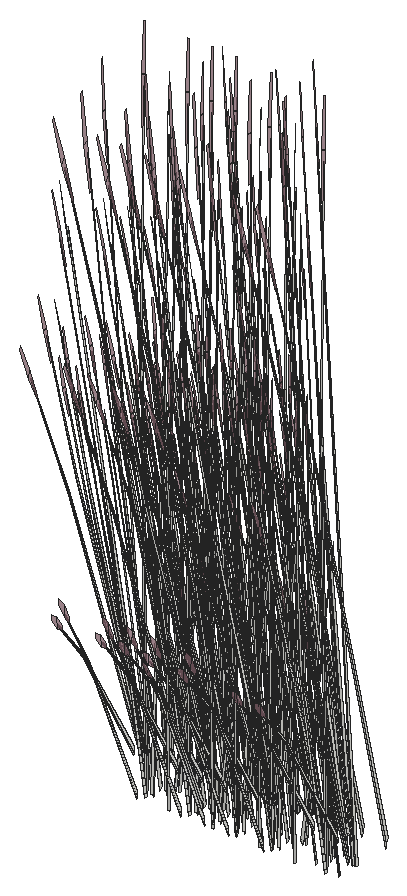
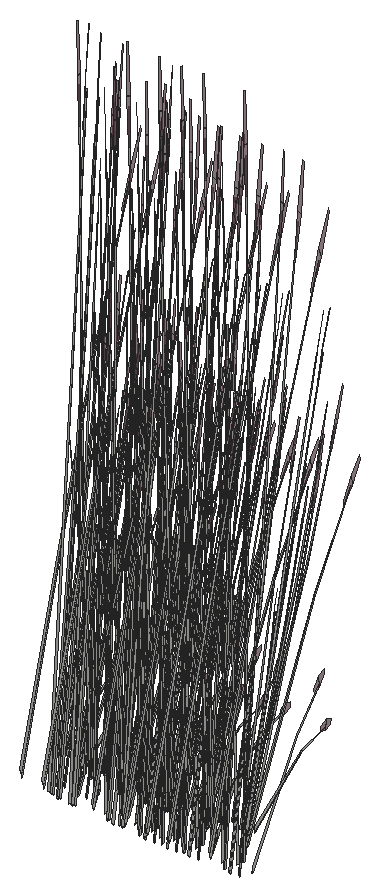
# SketchUp Ruby script. Lengths in inches.
U = 1.inch
M = Sketchup.active_model
def pt(a) = Geom::Point3d.new(a.map { |v| v * U })
def face(e, loops, mat)
  f = e.add_face(loops[0].map { |a| pt(a) })
  loops[1..].each { |l| e.add_face(l.map { |a| pt(a) }).erase! }
  f.material = f.back_material = mat if mat
  f
end
# faces: each face lists its corners as indices into pts; further lists are holes
def faces(e, pts, list, mat = nil) = list.each { |f| face(e, (f[0].is_a?(Array) ? f : [f]).map { |l| l.map { |i| pts[i] } }, mat) }
# xy, xz, yz: faces in a plane at the given z, y or x. An outline is a flat list of corners, or four numbers for a rectangle; further outlines are holes
def ring(l) = l.size == 4 ? [[l[0], l[1]], [l[2], l[1]], [l[2], l[3]], [l[0], l[3]]] : l.each_slice(2).to_a
def flat(e, list, mat, &to3) = list.each { |f| face(e, (f[0].is_a?(Array) ? f : [f]).map { |l| ring(l).map { |u, v| to3.(u, v) } }, mat) }
def xy(e, z, list, mat = nil) = flat(e, list, mat) { |x, y| [x, y, z] }
def xz(e, y, list, mat = nil) = flat(e, list, mat) { |x, z| [x, y, z] }
def yz(e, x, list, mat = nil) = flat(e, list, mat) { |y, z| [x, y, z] }
def lines(e, pts, list) = list.each { |a, b| e.add_line(pt(pts[a]), pt(pts[b])) }
# prism: a flat outline (further loops are holes) pulled along v
def prism(e, loops, v, mat = nil)
  f = face(e, loops, mat); d = Geom::Vector3d.new(v.map { |x| x * U })
  f.pushpull(f.normal.samedirection?(d) ? d.length : -d.length)
end
def box(e, o, s, mat = nil) = prism(e, [[o, [o[0] + s[0], o[1], o[2]], [o[0] + s[0], o[1] + s[1], o[2]], [o[0], o[1] + s[1], o[2]]]], [0, 0, s[2]], mat)
def at(x, y, z, deg = 0) = Geom::Transformation.translation(pt([x, y, z])) * Geom::Transformation.rotation(ORIGIN, Z_AXIS, deg.degrees)
def axes(o, x, y, z) = Geom::Transformation.new([*x, 0, *y, 0, *z, 0, *pt(o).to_a, 1])
def part(name) = M.definitions.add(name)
# library, detail: a bought-in or finely detailed component or shape, given as its bounding box
def library(name, o, s) = part(name).tap { |d| box(d.entities, o, s) }
def detail(e, o, s) = box(e.add_group.entities, o, s)
def put(e, d, t, mat = nil) = e.add_instance(d, t).tap { |i| i.material = mat if mat }
def group(e, t, mat = nil) = e.add_group.tap { |g| g.transformation = t; g.material = mat if mat }.entities
root = M.entities
M.materials.add("LightPink_Translucent").color = [144, 107, 117]
M.materials["LightPink_Translucent"].alpha = 0.75
c1 = part("blade")
p = [[2.15,0.21,22],[0,0.17,0],[0.09,0.45,0],[2.18,0.31,22],[2.29,0.31,22],[0.38,0.45,0],
  [2.48,0.24,33],[2.49,0.24,33],[2.48,0.22,33]]
faces(c1.entities,p,[[0,1,2,3],[4,5,2,3],[6,3,4,7],[8,0,3,6]])
c2 = part("seeds")
p = [[0.3,-0.1,1.38],[-0.01,-0.03,1.59],[-0.01,-0.03,0.03],[0.14,-0.07,-0.07],[0.29,-0.03,3],[0.15,0.01,3.11]]
faces(c2.entities,p,[[0,1,2,3],[1,0,4,5]],"LightPink_Translucent")
c3 = part("blade with seeds")
put(c3.entities,c1,at(0,0,0))
put(c3.entities,c2,axes([2.4,0.25,30.99],[1.5799,-0.05474,1.17369],[-0.12525,1.92788,0.29478],[-0.07173,-0.02425,1.56792]))
put(root,c3,axes([337,353.78,621.875],[0.1311,0.08035,1.71376],[-0.27131,0.33708,0.13857],[-0.16909,-0.15206,0.73262]))
put(root,c3,axes([336.97,353.04,622.72],[-0.07594,-0.00329,1.74944],[-0.24177,0.32918,-0.27667],[-0.129,-0.06726,0.14031]))
put(root,c3,axes([336.95,353.9,622.53],[-0.20082,-0.29199,-0.35414],[0.2293,-0.2764,0.4572],[-0.1165,-0.04206,0.87481]))
put(root,c3,axes([336.92,353.79,623.09],[0.29147,-0.34417,0.53763],[0.25138,0.3655,0.4433],[-0.13675,-0.06349,1.11249]))
put(root,c3,axes([337.05,353.79,622.73],[0.01777,-0.35463,0.0643],[0.26836,0.00972,0.50621],[-0.1028,-0.03711,0.77189]))
put(root,c3,axes([337.875,353.17,623.43],[-0.23555,0.44708,-0.13619],[-0.34112,-0.25757,-0.75594],[-0.11858,-0.12631,1.14864]))
put(root,c3,axes([337.77,353.54,622.98],[-0.30095,-0.22541,-0.71045],[0.21388,-0.395,0.08574],[-0.10904,-0.13459,1.00501]))
put(root,c3,axes([337.63,353.55,622.68],[-0.34827,0.11086,-0.51099],[-0.06092,-0.41983,-0.3958],[-0.09354,-0.12031,0.97773]))
put(root,c3,axes([337.18,353.16,619.49],[-0.03419,0.06144,1.76342],[-0.3455,0.13246,-0.26939],[-0.08346,-0.12049,0.30037]))
put(root,c3,axes([337.67,353.24,622.53],[-0.05451,-0.37564,-0.35414],[0.31161,-0.09919,0.4572],[-0.0837,-0.10765,0.87481]))
put(root,c3,axes([337.85,353.54,623.05],[0.05451,0.37564,0.35414],[-0.31161,0.09919,-0.4572],[-0.0837,-0.10765,0.87481]))
put(root,c3,axes([338.49,356.09,621.33],[0.305,0.18805,1.51261],[-0.29879,0.40513,0.59816],[-0.13384,-0.24012,1.26806]))
put(root,c3,axes([337.8,353.2,622.73],[0.16041,-0.29625,0.0643],[0.22843,0.17248,0.50621],[-0.07385,-0.09498,0.77189]))
put(root,c3,axes([336.9,354.79,620.02],[0,-0.46636,-0.49651],[0.39487,0,0],[0,-0.10622,1.57504]))
put(root,c3,axes([337.75,354.85,620.1],[-0.14494,-0.47823,-0.69835],[0.41752,-0.17223,-0.18329],[-0.01602,-0.16194,1.54149]))
put(root,c3,axes([338.18,352.91,620.13],[-0.2439,0.26754,-0.03893],[-0.22348,-0.29302,-0.17649],[-0.01573,-0.08303,0.58215]))
put(root,c3,axes([340.68,353.71,621.875],[0.1311,0.08035,1.71376],[-0.27131,0.33708,0.13857],[-0.16909,-0.15206,0.73262]))
put(root,c3,axes([338.6,353.48,623.05],[-0.1064,0.35863,0.35414],[-0.31043,-0.1046,-0.4572],[-0.02846,-0.14439,0.87481]))
put(root,c3,axes([340.65,352.97,622.72],[-0.07594,-0.00329,1.74944],[-0.24177,0.32918,-0.27667],[-0.129,-0.06726,0.14031]))
put(root,c3,axes([340.625,353.82,622.53],[-0.20082,-0.29199,-0.35414],[0.2293,-0.2764,0.4572],[-0.1165,-0.04206,0.87481]))
put(root,c3,axes([337.97,354.98,620.21],[0.17124,-0.42022,-0.44739],[0.35581,0.20224,0.21531],[0,-0.09687,1.43643]))
put(root,c3,axes([340.59,353.71,623.09],[0.29147,-0.34417,0.53763],[0.25138,0.3655,0.4433],[-0.13675,-0.06349,1.11249]))
put(root,c3,axes([338.69,353.16,622.73],[0.26007,-0.1585,0.0643],[0.12729,0.28902,0.50621],[-0.02512,-0.1274,0.77189]))
put(root,c3,axes([340.73,353.71,622.73],[0.01777,-0.35463,0.0643],[0.26836,0.00972,0.50621],[-0.1028,-0.03711,0.77189]))
put(root,c3,axes([337.7,353.48,620.375],[-0.22066,-0.46731,0],[0.36918,-0.26061,-0.51607],[0.08408,-0.05936,1.63711]))
put(root,c3,axes([341.55,353.09,623.43],[-0.23555,0.44708,-0.13619],[-0.34112,-0.25757,-0.75594],[-0.11858,-0.12631,1.14864]))
put(root,c3,axes([341.31,353.47,622.68],[-0.34827,0.11086,-0.51099],[-0.06092,-0.41983,-0.3958],[-0.09354,-0.12031,0.97773]))
put(root,c3,axes([340.86,353.09,619.49],[-0.03419,0.06144,1.76342],[-0.3455,0.13246,-0.26939],[-0.08346,-0.12049,0.30037]))
put(root,c3,axes([339.27,353.89,623.05],[-0.23881,0.24554,0.35414],[-0.22606,-0.28036,-0.4572],[0.0344,-0.14245,0.87481]))
put(root,c3,axes([342.55,353.81,621.875],[0.1311,0.08035,1.71376],[-0.27131,0.33708,0.13857],[-0.16909,-0.15206,0.73262]))
put(root,c3,axes([338,353.41,620.02],[0.33032,-0.23318,-0.49651],[0.19744,0.41812,0],[0.07523,-0.05311,1.57504]))
put(root,c3,axes([342.52,353.07,622.72],[-0.07594,-0.00329,1.74944],[-0.24177,0.32918,-0.27667],[-0.129,-0.06726,0.14031]))
put(root,c3,axes([341.53,353.47,623.05],[0.05451,0.37564,0.35414],[-0.31161,0.09919,-0.4572],[-0.0837,-0.10765,0.87481]))
put(root,c3,axes([342.17,356.01,621.33],[0.305,0.18805,1.51261],[-0.29879,0.40513,0.59816],[-0.13384,-0.24012,1.26806]))
put(root,c3,axes([341.48,353.125,622.73],[0.16041,-0.29625,0.0643],[0.22843,0.17248,0.50621],[-0.07385,-0.09498,0.77189]))
put(root,c3,axes([339.48,353.67,622.73],[0.29004,0.02173,0.0643],[-0.00795,0.32812,0.50621],[0.03035,-0.12569,0.77189]))
put(root,c3,axes([342.47,353.8125,623.09],[0.29147,-0.34417,0.53763],[0.25138,0.3655,0.4433],[-0.13675,-0.06349,1.11249]))
put(root,c3,axes([338.39,354.36,620.06],[0.23773,-0.35053,-0.62353],[0.29532,0.31785,-0.16365],[0.09526,-0.08744,1.37633]))
put(root,c3,axes([339.39,353.64,622.73],[0.25132,0.3182,0.48003],[-0.2669,0.27442,0.3958],[0.04636,-0.14929,0.9933]))
put(root,c3,axes([340.58,354.71,620.02],[0,-0.46636,-0.49651],[0.39487,0,0],[0,-0.10622,1.57504]))
put(root,c3,axes([342.6,353.81,622.73],[0.01777,-0.35463,0.0643],[0.26836,0.00972,0.50621],[-0.1028,-0.03711,0.77189]))
put(root,c3,axes([343.42,353.2,623.43],[-0.23555,0.44708,-0.13619],[-0.34112,-0.25757,-0.75594],[-0.11858,-0.12631,1.14864]))
put(root,c3,axes([343.32,353.56,622.98],[-0.30095,-0.22541,-0.71045],[0.21388,-0.395,0.08574],[-0.10904,-0.13459,1.00501]))
put(root,c3,axes([343.18,353.57,622.68],[-0.34827,0.11086,-0.51099],[-0.06092,-0.41983,-0.3958],[-0.09354,-0.12031,0.97773]))
put(root,c3,axes([341.43,354.78,620.1],[-0.14494,-0.47823,-0.69835],[0.41752,-0.17223,-0.18329],[-0.01602,-0.16194,1.54149]))
put(root,c3,axes([339.84,354.68,623.03],[-0.32648,-0.25715,-0.1216],[0.18809,-0.3724,-0.67495],[0.09224,-0.12945,1.02557]))
put(root,c3,axes([342.73,353.1875,619.49],[-0.03419,0.06144,1.76342],[-0.3455,0.13246,-0.26939],[-0.08346,-0.12049,0.30037]))
put(root,c3,axes([341.86,352.84,620.13],[-0.2439,0.26754,-0.03893],[-0.22348,-0.29302,-0.17649],[-0.01573,-0.08303,0.58215]))
put(root,c3,axes([339.69,353.39,619.49],[-0.05283,-0.03674,1.76342],[-0.13569,-0.41045,-0.26939],[0.09154,-0.11138,0.30037]))
put(root,c3,axes([339.68,354.38,622.68],[-0.09067,-0.42583,-0.51099],[0.34336,-0.07449,-0.3958],[0.0984,-0.11438,0.97773]))
put(root,c3,axes([342.28,353.41,623.05],[-0.1064,0.35863,0.35414],[-0.31043,-0.1046,-0.4572],[-0.02846,-0.14439,0.87481]))
put(root,c3,axes([344.59,353.72,621.875],[0.1311,0.08035,1.71376],[-0.27131,0.33708,0.13857],[-0.16909,-0.15206,0.73262]))
put(root,c3,axes([340.1,353.53,620.77],[-0.11756,0.2374,1.1486],[-0.10105,-0.31895,0.84392],[0.09709,-0.07992,0.25299]))
put(root,c3,axes([343.22,353.26,622.53],[-0.05451,-0.37564,-0.35414],[0.31161,-0.09919,0.4572],[-0.0837,-0.10765,0.87481]))
put(root,c3,axes([343.4,353.57,623.05],[0.05451,0.37564,0.35414],[-0.31161,0.09919,-0.4572],[-0.0837,-0.10765,0.87481]))
put(root,c3,axes([340.64,354.57,622.71],[-0.0461,-0.00354,1.77383],[-0.19143,-0.37951,-0.16761],[0.07688,-0.12478,0.31391]))
put(root,c3,axes([341.65,354.9,620.21],[0.17124,-0.42022,-0.44739],[0.35581,0.20224,0.21531],[0,-0.09687,1.43643]))
put(root,c3,axes([339.93,354.42,622.53],[0.30722,-0.06665,-0.35414],[0.08112,0.381,0.4572],[0.08804,-0.10234,0.87481]))
put(root,c3,axes([344.04,356.11,621.33],[0.305,0.18805,1.51261],[-0.29879,0.40513,0.59816],[-0.13384,-0.24012,1.26806]))
put(root,c3,axes([339.6875,354.55,622.98],[0.18436,-0.36797,-0.71045],[0.32306,0.26151,0.08574],[0.11008,-0.13332,1.00501]))
put(root,c3,axes([342.88,352.7,620.77],[0.18411,0.16231,1.1486],[-0.26813,0.09757,0.84392],[-0.05737,-0.12474,0.25299]))
put(root,c3,axes([344.57,352.98,622.72],[-0.07594,-0.00329,1.74944],[-0.24177,0.32918,-0.27667],[-0.129,-0.06726,0.14031]))
put(root,c3,axes([344.54,353.83,622.53],[-0.20082,-0.29199,-0.35414],[0.2293,-0.2764,0.4572],[-0.1165,-0.04206,0.87481]))
put(root,c3,axes([343.35,353.23,622.73],[0.16041,-0.29625,0.0643],[0.22843,0.17248,0.50621],[-0.07385,-0.09498,0.77189]))
put(root,c3,axes([344.51,353.72,623.09],[0.29147,-0.34417,0.53763],[0.25138,0.3655,0.4433],[-0.13675,-0.06349,1.11249]))
put(root,c3,axes([342.45,354.81,620.02],[0,-0.46636,-0.49651],[0.39487,0,0],[0,-0.10622,1.57504]))
put(root,c3,axes([339.96,354.21,620.59],[-0.12609,-0.01381,1.43002],[-0.12917,-0.37055,-0.30754],[0.1549,-0.10482,0.61141]))
put(root,c3,axes([341.375,353.4,620.375],[-0.22066,-0.46731,0],[0.36918,-0.26061,-0.51607],[0.08408,-0.05936,1.63711]))
put(root,c3,axes([344.64,353.72,622.73],[0.01777,-0.35463,0.0643],[0.26836,0.00972,0.50621],[-0.1028,-0.03711,0.77189]))
put(root,c3,axes([343.3,354.875,620.1],[-0.14494,-0.47823,-0.69835],[0.41752,-0.17223,-0.18329],[-0.01602,-0.16194,1.54149]))
put(root,c3,axes([345.47,353.11,623.43],[-0.23555,0.44708,-0.13619],[-0.34112,-0.25757,-0.75594],[-0.11858,-0.12631,1.14864]))
put(root,c3,axes([345.23,353.48,622.68],[-0.34827,0.11086,-0.51099],[-0.06092,-0.41983,-0.3958],[-0.09354,-0.12031,0.97773]))
put(root,c3,axes([343.73,352.9375,620.13],[-0.2439,0.26754,-0.03893],[-0.22348,-0.29302,-0.17649],[-0.01573,-0.08303,0.58215]))
put(root,c3,axes([344.78,353.1,619.49],[-0.03419,0.06144,1.76342],[-0.3455,0.13246,-0.26939],[-0.08346,-0.12049,0.30037]))
put(root,c3,axes([342.95,353.81,623.05],[-0.23881,0.24554,0.35414],[-0.22606,-0.28036,-0.4572],[0.0344,-0.14245,0.87481]))
put(root,c3,axes([341.81,354.69,620.67],[-0.04113,-0.53214,-0.29095],[0.42835,-0.03218,-0.50002],[0.07543,-0.07088,1.59708]))
put(root,c3,axes([344.15,353.51,623.05],[-0.1064,0.35863,0.35414],[-0.31043,-0.1046,-0.4572],[-0.02846,-0.14439,0.87481]))
put(root,c3,axes([341.67,353.33,620.02],[0.33032,-0.23318,-0.49651],[0.19744,0.41812,0],[0.07523,-0.05311,1.57504]))
put(root,c3,axes([345.45,353.48,623.05],[0.05451,0.37564,0.35414],[-0.31161,0.09919,-0.4572],[-0.0837,-0.10765,0.87481]))
put(root,c3,axes([346.09,356.02,621.33],[0.305,0.18805,1.51261],[-0.29879,0.40513,0.59816],[-0.13384,-0.24012,1.26806]))
put(root,c3,axes([343.16,353.59,622.73],[0.29004,0.02173,0.0643],[-0.00795,0.32812,0.50621],[0.03035,-0.12569,0.77189]))
put(root,c3,axes([344.24,353.18,622.73],[0.26007,-0.1585,0.0643],[0.12729,0.28902,0.50621],[-0.02512,-0.1274,0.77189]))
put(root,c3,axes([342.06,354.28,620.06],[0.23773,-0.35053,-0.62353],[0.29532,0.31785,-0.16365],[0.09526,-0.08744,1.37633]))
put(root,c3,axes([343.07,353.56,622.73],[0.25132,0.3182,0.48003],[-0.2669,0.27442,0.3958],[0.04636,-0.14929,0.9933]))
put(root,c3,axes([345.4,353.14,622.73],[0.16041,-0.29625,0.0643],[0.22843,0.17248,0.50621],[-0.07385,-0.09498,0.77189]))
put(root,c3,axes([343.24,353.5,620.375],[-0.22066,-0.46731,0],[0.36918,-0.26061,-0.51607],[0.08408,-0.05936,1.63711]))
put(root,c3,axes([344.49,354.72,620.02],[0,-0.46636,-0.49651],[0.39487,0,0],[0,-0.10622,1.57504]))
put(root,c3,axes([347.53,353.89,620.59],[0.06891,0.12984,1.43002],[-0.15879,0.35293,-0.30754],[-0.16304,-0.08436,0.61141]))
put(root,c3,axes([347.66,353.47,621.875],[0.1311,0.08035,1.71376],[-0.27131,0.33708,0.13857],[-0.16909,-0.15206,0.73262]))
put(root,c3,axes([343.52,354.6,623.03],[-0.32648,-0.25715,-0.1216],[0.18809,-0.3724,-0.67495],[0.09224,-0.12945,1.02557]))
put(root,c3,axes([343.37,353.3125,619.49],[-0.05283,-0.03674,1.76342],[-0.13569,-0.41045,-0.26939],[0.09154,-0.11138,0.30037]))
put(root,c3,axes([345.35,354.79,620.1],[-0.14494,-0.47823,-0.69835],[0.41752,-0.17223,-0.18329],[-0.01602,-0.16194,1.54149]))
put(root,c3,axes([344.82,353.91,623.05],[-0.23881,0.24554,0.35414],[-0.22606,-0.28036,-0.4572],[0.0344,-0.14245,0.87481]))
put(root,c3,axes([343.36,354.3,622.68],[-0.09067,-0.42583,-0.51099],[0.34336,-0.07449,-0.3958],[0.0984,-0.11438,0.97773]))
put(root,c3,axes([345.77,352.85,620.13],[-0.2439,0.26754,-0.03893],[-0.22348,-0.29302,-0.17649],[-0.01573,-0.08303,0.58215]))
put(root,c3,axes([347.63,352.73,622.72],[-0.07594,-0.00329,1.74944],[-0.24177,0.32918,-0.27667],[-0.129,-0.06726,0.14031]))
put(root,c3,axes([347.61,353.58,622.53],[-0.20082,-0.29199,-0.35414],[0.2293,-0.2764,0.4572],[-0.1165,-0.04206,0.87481]))
put(root,c3,axes([343.78,353.45,620.77],[-0.11756,0.2374,1.1486],[-0.10105,-0.31895,0.84392],[0.09709,-0.07992,0.25299]))
put(root,c3,axes([343.54,353.43,620.02],[0.33032,-0.23318,-0.49651],[0.19744,0.41812,0],[0.07523,-0.05311,1.57504]))
put(root,c3,axes([346.19,353.42,623.05],[-0.1064,0.35863,0.35414],[-0.31043,-0.1046,-0.4572],[-0.02846,-0.14439,0.87481]))
put(root,c3,axes([347.58,353.47,623.09],[0.29147,-0.34417,0.53763],[0.25138,0.3655,0.4433],[-0.13675,-0.06349,1.11249]))
put(root,c3,axes([344.32,354.49,622.71],[-0.0461,-0.00354,1.77383],[-0.19143,-0.37951,-0.16761],[0.07688,-0.12478,0.31391]))
put(root,c3,axes([343.61,354.34,622.53],[0.30722,-0.06665,-0.35414],[0.08112,0.381,0.4572],[0.08804,-0.10234,0.87481]))
put(root,c3,axes([343.37,354.47,622.98],[0.18436,-0.36797,-0.71045],[0.32306,0.26151,0.08574],[0.11008,-0.13332,1.00501]))
put(root,c3,axes([345.57,354.91,620.21],[0.17124,-0.42022,-0.44739],[0.35581,0.20224,0.21531],[0,-0.09687,1.43643]))
put(root,c3,axes([347.71,353.47,622.73],[0.01777,-0.35463,0.0643],[0.26836,0.00972,0.50621],[-0.1028,-0.03711,0.77189]))
put(root,c3,axes([344.94,353.5625,622.53],[0.23881,-0.24554,-0.35414],[0.22606,0.28036,0.4572],[0.0344,-0.14245,0.87481]))
put(root,c3,axes([348.53,352.85,623.43],[-0.23555,0.44708,-0.13619],[-0.34112,-0.25757,-0.75594],[-0.11858,-0.12631,1.14864]))
put(root,c3,axes([345.03,353.6875,622.73],[0.29004,0.02173,0.0643],[-0.00795,0.32812,0.50621],[0.03035,-0.12569,0.77189]))
put(root,c3,axes([343.9375,354.38,620.06],[0.23773,-0.35053,-0.62353],[0.29532,0.31785,-0.16365],[0.09526,-0.08744,1.37633]))
put(root,c3,axes([348.29,353.23,622.68],[-0.34827,0.11086,-0.51099],[-0.06092,-0.41983,-0.3958],[-0.09354,-0.12031,0.97773]))
put(root,c3,axes([344.94,353.66,622.73],[0.25132,0.3182,0.48003],[-0.2669,0.27442,0.3958],[0.04636,-0.14929,0.9933]))
put(root,c3,axes([347.84,352.85,619.49],[-0.03419,0.06144,1.76342],[-0.3455,0.13246,-0.26939],[-0.08346,-0.12049,0.30037]))
put(root,c3,axes([343.63,354.13,620.59],[-0.12609,-0.01381,1.43002],[-0.12917,-0.37055,-0.30754],[0.1549,-0.10482,0.61141]))
put(root,c3,axes([347.625,353.08,620.13],[-0.10181,0.3808,-0.03893],[-0.31336,-0.11714,-0.17649],[-0.04758,-0.06228,0.58215]))
put(root,c3,axes([345.29,353.41,620.375],[-0.22066,-0.46731,0],[0.36918,-0.26061,-0.51607],[0.08408,-0.05936,1.63711]))
put(root,c3,axes([345.39,354.7,623.03],[-0.32648,-0.25715,-0.1216],[0.18809,-0.3724,-0.67495],[0.09224,-0.12945,1.02557]))
put(root,c3,axes([345.24,353.41,619.49],[-0.05283,-0.03674,1.76342],[-0.13569,-0.41045,-0.26939],[0.09154,-0.11138,0.30037]))
put(root,c3,axes([347.46,354.82,620.375],[-0.44133,0,0],[0,-0.52122,-0.51607],[0,-0.11871,1.63711]))
put(root,c3,axes([345.23,354.4,622.68],[-0.09067,-0.42583,-0.51099],[0.34336,-0.07449,-0.3958],[0.0984,-0.11438,0.97773]))
put(root,c3,axes([348.51,353.23,623.05],[0.05451,0.37564,0.35414],[-0.31161,0.09919,-0.4572],[-0.0837,-0.10765,0.87481]))
put(root,c3,axes([346.86,353.82,623.05],[-0.23881,0.24554,0.35414],[-0.22606,-0.28036,-0.4572],[0.0344,-0.14245,0.87481]))
put(root,c3,axes([349.15,355.77,621.33],[0.305,0.18805,1.51261],[-0.29879,0.40513,0.59816],[-0.13384,-0.24012,1.26806]))
put(root,c3,axes([345.72,354.7,620.67],[-0.04113,-0.53214,-0.29095],[0.42835,-0.03218,-0.50002],[0.07543,-0.07088,1.59708]))
put(root,c3,axes([345.65,353.55,620.77],[-0.11756,0.2374,1.1486],[-0.10105,-0.31895,0.84392],[0.09709,-0.07992,0.25299]))
put(root,c3,axes([348.46,352.89,622.73],[0.16041,-0.29625,0.0643],[0.22843,0.17248,0.50621],[-0.07385,-0.09498,0.77189]))
put(root,c3,axes([345.59,353.34,620.02],[0.33032,-0.23318,-0.49651],[0.19744,0.41812,0],[0.07523,-0.05311,1.57504]))
put(root,c3,axes([346.19,354.59,622.71],[-0.0461,-0.00354,1.77383],[-0.19143,-0.37951,-0.16761],[0.07688,-0.12478,0.31391]))
put(root,c3,axes([345.48,354.44,622.53],[0.30722,-0.06665,-0.35414],[0.08112,0.381,0.4572],[0.08804,-0.10234,0.87481]))
put(root,c3,axes([345.24,354.57,622.98],[0.18436,-0.36797,-0.71045],[0.32306,0.26151,0.08574],[0.11008,-0.13332,1.00501]))
put(root,c3,axes([347.56,354.47,620.02],[0,-0.46636,-0.49651],[0.39487,0,0],[0,-0.10622,1.57504]))
put(root,c3,axes([348.59,355.01,620.67],[-0.39748,-0.22252,-0.29095],[0.19139,-0.46966,-0.50002],[-0.01249,-0.11531,1.59708]))
put(root,c3,axes([348.41,354.54,620.1],[-0.14494,-0.47823,-0.69835],[0.41752,-0.17223,-0.18329],[-0.01602,-0.16194,1.54149]))
put(root,c3,axes([347.08,353.6,622.73],[0.29004,0.02173,0.0643],[-0.00795,0.32812,0.50621],[0.03035,-0.12569,0.77189]))
put(root,c3,axes([345.5,354.23,620.59],[-0.12609,-0.01381,1.43002],[-0.12917,-0.37055,-0.30754],[0.1549,-0.10482,0.61141]))
put(root,c3,axes([345.98,354.29,620.06],[0.23773,-0.35053,-0.62353],[0.29532,0.31785,-0.16365],[0.09526,-0.08744,1.37633]))
put(root,c3,axes([346.99,353.57,622.73],[0.25132,0.3182,0.48003],[-0.2669,0.27442,0.3958],[0.04636,-0.14929,0.9933]))
put(root,c3,axes([347.73,354.48,620.03],[0.24637,-0.29097,-0.30978],[0.24637,0.29097,0.30978],[0,-0.09372,1.38974]))
put(root,c3,axes([348.84,352.6,620.13],[-0.2439,0.26754,-0.03893],[-0.22348,-0.29302,-0.17649],[-0.01573,-0.08303,0.58215]))
put(root,c3,axes([349.26,353.17,623.05],[-0.1064,0.35863,0.35414],[-0.31043,-0.1046,-0.4572],[-0.02846,-0.14439,0.87481]))
put(root,c3,axes([347.44,354.61,623.03],[-0.32648,-0.25715,-0.1216],[0.18809,-0.3724,-0.67495],[0.09224,-0.12945,1.02557]))
put(root,c3,axes([347.28,353.32,619.49],[-0.05283,-0.03674,1.76342],[-0.13569,-0.41045,-0.26939],[0.09154,-0.11138,0.30037]))
put(root,c3,axes([348.63,354.66,620.21],[0.17124,-0.42022,-0.44739],[0.35581,0.20224,0.21531],[0,-0.09687,1.43643]))
put(root,c3,axes([347.27,354.31,622.68],[-0.09067,-0.42583,-0.51099],[0.34336,-0.07449,-0.3958],[0.0984,-0.11438,0.97773]))
put(root,c3,axes([352.41,353.54,622.98],[-0.35281,-0.01123,-0.71045],[0.0237,-0.47284,0.08574],[-0.14947,-0.0499,1.00501]))
put(root,c3,axes([352.125,353.66,620.59],[0.06891,0.12984,1.43002],[-0.15879,0.35293,-0.30754],[-0.16304,-0.08436,0.61141]))
put(root,c3,axes([347.69,353.46,620.77],[-0.11756,0.2374,1.1486],[-0.10105,-0.31895,0.84392],[0.09709,-0.07992,0.25299]))
put(root,c3,axes([348.24,354.5,622.71],[-0.0461,-0.00354,1.77383],[-0.19143,-0.37951,-0.16761],[0.07688,-0.12478,0.31391]))
put(root,c3,axes([347.53,354.35,622.53],[0.30722,-0.06665,-0.35414],[0.08112,0.381,0.4572],[0.08804,-0.10234,0.87481]))
put(root,c3,axes([347.28,354.48,622.98],[0.18436,-0.36797,-0.71045],[0.32306,0.26151,0.08574],[0.11008,-0.13332,1.00501]))
put(root,c3,axes([348.35,353.16,620.375],[-0.22066,-0.46731,0],[0.36918,-0.26061,-0.51607],[0.08408,-0.05936,1.63711]))
put(root,c3,axes([352.22,352.49,622.72],[-0.07594,-0.00329,1.74944],[-0.24177,0.32918,-0.27667],[-0.129,-0.06726,0.14031]))
put(root,c3,axes([352.2,353.35,622.53],[-0.20082,-0.29199,-0.35414],[0.2293,-0.2764,0.4572],[-0.1165,-0.04206,0.87481]))
put(root,c3,axes([347.55,354.14,620.59],[-0.12609,-0.01381,1.43002],[-0.12917,-0.37055,-0.30754],[0.1549,-0.10482,0.61141]))
put(root,c3,axes([349.93,353.57,623.05],[-0.23881,0.24554,0.35414],[-0.22606,-0.28036,-0.4572],[0.0344,-0.14245,0.87481]))
put(root,c3,axes([352.17,353.24,623.09],[0.29147,-0.34417,0.53763],[0.25138,0.3655,0.4433],[-0.13675,-0.06349,1.11249]))
put(root,c3,axes([348.79,354.45,620.67],[-0.04113,-0.53214,-0.29095],[0.42835,-0.03218,-0.50002],[0.07543,-0.07088,1.59708]))
put(root,c3,axes([352.3,353.23,622.73],[0.01777,-0.35463,0.0643],[0.26836,0.00972,0.50621],[-0.1028,-0.03711,0.77189]))
put(root,c3,axes([348.65,353.09,620.02],[0.33032,-0.23318,-0.49651],[0.19744,0.41812,0],[0.07523,-0.05311,1.57504]))
put(root,c3,axes([353.13,352.62,623.43],[-0.23555,0.44708,-0.13619],[-0.34112,-0.25757,-0.75594],[-0.11858,-0.12631,1.14864]))
put(root,c3,axes([352.88,353,622.68],[-0.34827,0.11086,-0.51099],[-0.06092,-0.41983,-0.3958],[-0.09354,-0.12031,0.97773]))
put(root,c3,axes([350.14,353.35,622.73],[0.29004,0.02173,0.0643],[-0.00795,0.32812,0.50621],[0.03035,-0.12569,0.77189]))
put(root,c3,axes([352.22,352.85,620.13],[-0.10181,0.3808,-0.03893],[-0.31336,-0.11714,-0.17649],[-0.04758,-0.06228,0.58215]))
put(root,c3,axes([349.05,354.04,620.06],[0.23773,-0.35053,-0.62353],[0.29532,0.31785,-0.16365],[0.09526,-0.08744,1.37633]))
put(root,c3,axes([350.05,353.32,622.73],[0.25132,0.3182,0.48003],[-0.2669,0.27442,0.3958],[0.04636,-0.14929,0.9933]))
put(root,c3,axes([354.57,353.27,622.98],[-0.35281,-0.01123,-0.71045],[0.0237,-0.47284,0.08574],[-0.14947,-0.0499,1.00501]))
put(root,c3,axes([354.28,353.38,620.59],[0.06891,0.12984,1.43002],[-0.15879,0.35293,-0.30754],[-0.16304,-0.08436,0.61141]))
put(root,c3,axes([352.05,354.59,620.375],[-0.44133,0,0],[0,-0.52122,-0.51607],[0,-0.11871,1.63711]))
put(root,c3,axes([350.34,354.33,623.05],[-0.30722,0.06665,0.35414],[-0.08112,-0.381,-0.4572],[0.08804,-0.10234,0.87481]))
put(root,c3,axes([353.1,352.99,623.05],[0.05451,0.37564,0.35414],[-0.31161,0.09919,-0.4572],[-0.0837,-0.10765,0.87481]))
put(root,c3,axes([353.74,355.53,621.33],[0.305,0.18805,1.51261],[-0.29879,0.40513,0.59816],[-0.13384,-0.24012,1.26806]))
put(root,c3,axes([350.5,354.36,623.03],[-0.32648,-0.25715,-0.1216],[0.18809,-0.3724,-0.67495],[0.09224,-0.12945,1.02557]))
put(root,c3,axes([354.38,352.22,622.72],[-0.07594,-0.00329,1.74944],[-0.24177,0.32918,-0.27667],[-0.129,-0.06726,0.14031]))
put(root,c3,axes([350.35,353.07,619.49],[-0.05283,-0.03674,1.76342],[-0.13569,-0.41045,-0.26939],[0.09154,-0.11138,0.30037]))
put(root,c3,axes([354.36,353.07,622.53],[-0.20082,-0.29199,-0.35414],[0.2293,-0.2764,0.4572],[-0.1165,-0.04206,0.87481]))
put(root,c3,axes([350.34,354.06,622.68],[-0.09067,-0.42583,-0.51099],[0.34336,-0.07449,-0.3958],[0.0984,-0.11438,0.97773]))
put(root,c3,axes([352.15,354.23,620.02],[0,-0.46636,-0.49651],[0.39487,0,0],[0,-0.10622,1.57504]))
put(root,c3,axes([354.33,352.96,623.09],[0.29147,-0.34417,0.53763],[0.25138,0.3655,0.4433],[-0.13675,-0.06349,1.11249]))
put(root,c3,axes([350.76,353.21,620.77],[-0.11756,0.2374,1.1486],[-0.10105,-0.31895,0.84392],[0.09709,-0.07992,0.25299]))
put(root,c3,axes([353.18,354.77,620.67],[-0.39748,-0.22252,-0.29095],[0.19139,-0.46966,-0.50002],[-0.01249,-0.11531,1.59708]))
put(root,c3,axes([351.3,354.25,622.71],[-0.0461,-0.00354,1.77383],[-0.19143,-0.37951,-0.16761],[0.07688,-0.12478,0.31391]))
put(root,c3,axes([350.59,354.1,622.53],[0.30722,-0.06665,-0.35414],[0.08112,0.381,0.4572],[0.08804,-0.10234,0.87481]))
put(root,c3,axes([350.35,354.23,622.98],[0.18436,-0.36797,-0.71045],[0.32306,0.26151,0.08574],[0.11008,-0.13332,1.00501]))
put(root,c3,axes([354.46,352.96,622.73],[0.01777,-0.35463,0.0643],[0.26836,0.00972,0.50621],[-0.1028,-0.03711,0.77189]))
put(root,c3,axes([352.32,354.24,620.03],[0.24637,-0.29097,-0.30978],[0.24637,0.29097,0.30978],[0,-0.09372,1.38974]))
put(root,c3,axes([353.43,352.36,620.13],[-0.2439,0.26754,-0.03893],[-0.22348,-0.29302,-0.17649],[-0.01573,-0.08303,0.58215]))
put(root,c3,axes([353.85,352.93,623.05],[-0.1064,0.35863,0.35414],[-0.31043,-0.1046,-0.4572],[-0.02846,-0.14439,0.87481]))
put(root,c3,axes([350.61,353.89,620.59],[-0.12609,-0.01381,1.43002],[-0.12917,-0.37055,-0.30754],[0.1549,-0.10482,0.61141]))
put(root,c3,axes([354.375,352.58,620.13],[-0.10181,0.3808,-0.03893],[-0.31336,-0.11714,-0.17649],[-0.04758,-0.06228,0.58215]))
put(root,c3,axes([353.22,354.42,620.21],[0.17124,-0.42022,-0.44739],[0.35581,0.20224,0.21531],[0,-0.09687,1.43643]))
put(root,c3,axes([354.21,354.3125,620.375],[-0.44133,0,0],[0,-0.52122,-0.51607],[0,-0.11871,1.63711]))
put(root,c3,axes([355.26,352.72,623.05],[0.05451,0.37564,0.35414],[-0.31161,0.09919,-0.4572],[-0.0837,-0.10765,0.87481]))
put(root,c3,axes([354.55,354.18,620.33],[-0.32829,0.39208,0.30756],[-0.32849,-0.38796,-0.36492],[-0.01146,-0.11134,1.64885]))
put(root,c3,axes([355.9,355.26,621.33],[0.305,0.18805,1.51261],[-0.29879,0.40513,0.59816],[-0.13384,-0.24012,1.26806]))
put(root,c3,axes([352.95,352.93,620.375],[-0.22066,-0.46731,0],[0.36918,-0.26061,-0.51607],[0.08408,-0.05936,1.63711]))
